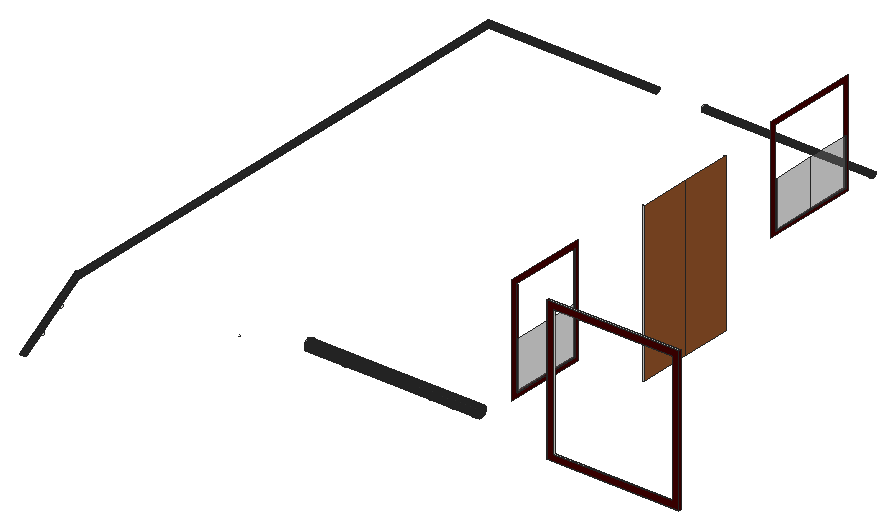
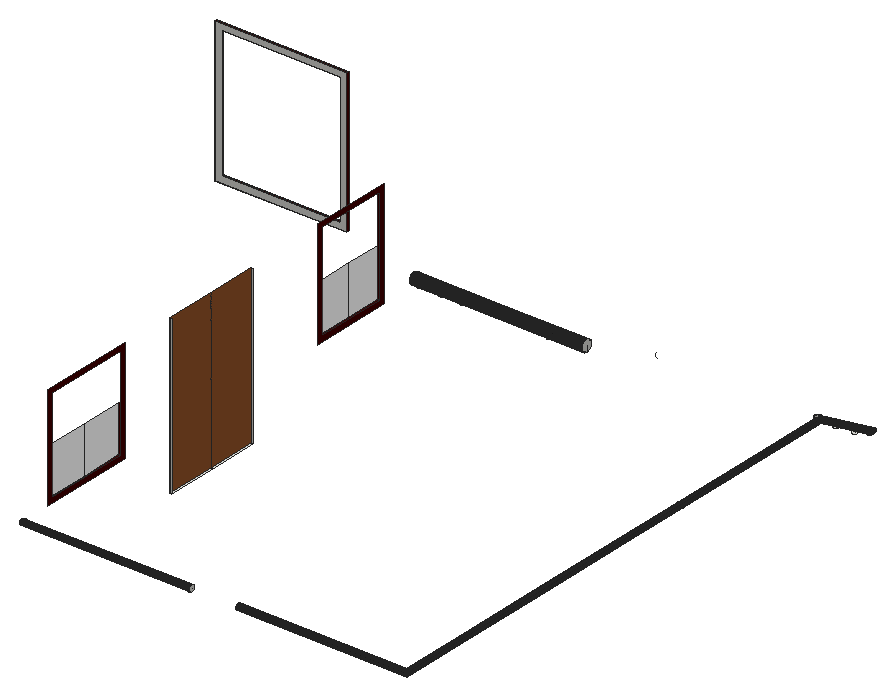
# SketchUp Ruby script. Lengths in inches.
U = 1.inch
M = Sketchup.active_model
def pt(a) = Geom::Point3d.new(a.map { |v| v * U })
def face(e, loops, mat)
  f = e.add_face(loops[0].map { |a| pt(a) })
  loops[1..].each { |l| e.add_face(l.map { |a| pt(a) }).erase! }
  f.material = f.back_material = mat if mat
  f
end
# faces: each face lists its corners as indices into pts; further lists are holes
def faces(e, pts, list, mat = nil) = list.each { |f| face(e, (f[0].is_a?(Array) ? f : [f]).map { |l| l.map { |i| pts[i] } }, mat) }
# xy, xz, yz: faces in a plane at the given z, y or x. An outline is a flat list of corners, or four numbers for a rectangle; further outlines are holes
def ring(l) = l.size == 4 ? [[l[0], l[1]], [l[2], l[1]], [l[2], l[3]], [l[0], l[3]]] : l.each_slice(2).to_a
def flat(e, list, mat, &to3) = list.each { |f| face(e, (f[0].is_a?(Array) ? f : [f]).map { |l| ring(l).map { |u, v| to3.(u, v) } }, mat) }
def xy(e, z, list, mat = nil) = flat(e, list, mat) { |x, y| [x, y, z] }
def xz(e, y, list, mat = nil) = flat(e, list, mat) { |x, z| [x, y, z] }
def yz(e, x, list, mat = nil) = flat(e, list, mat) { |y, z| [x, y, z] }
def lines(e, pts, list) = list.each { |a, b| e.add_line(pt(pts[a]), pt(pts[b])) }
# prism: a flat outline (further loops are holes) pulled along v
def prism(e, loops, v, mat = nil)
  f = face(e, loops, mat); d = Geom::Vector3d.new(v.map { |x| x * U })
  f.pushpull(f.normal.samedirection?(d) ? d.length : -d.length)
end
def box(e, o, s, mat = nil) = prism(e, [[o, [o[0] + s[0], o[1], o[2]], [o[0] + s[0], o[1] + s[1], o[2]], [o[0], o[1] + s[1], o[2]]]], [0, 0, s[2]], mat)
def at(x, y, z, deg = 0) = Geom::Transformation.translation(pt([x, y, z])) * Geom::Transformation.rotation(ORIGIN, Z_AXIS, deg.degrees)
def axes(o, x, y, z) = Geom::Transformation.new([*x, 0, *y, 0, *z, 0, *pt(o).to_a, 1])
def part(name) = M.definitions.add(name)
# library, detail: a bought-in or finely detailed component or shape, given as its bounding box
def library(name, o, s) = part(name).tap { |d| box(d.entities, o, s) }
def detail(e, o, s) = box(e.add_group.entities, o, s)
def put(e, d, t, mat = nil) = e.add_instance(d, t).tap { |i| i.material = mat if mat }
def group(e, t, mat = nil) = e.add_group.tap { |g| g.transformation = t; g.material = mat if mat }.entities
root = M.entities
M.materials.add("[0022_Maroon]").color = [68, 0, 0]
M.materials.add("[0137_Black]").color = [45, 45, 45]
M.materials.add("[Translucent Glass Gray]").color = [128, 128, 128]
M.materials["[Translucent Glass Gray]"].alpha = 0.5
M.materials.add("[Wood Cherry Original]").color = [152, 86, 42]
xy(root,53.06,[[432,334.98,434,391.49],[432,391.49,434,447.99]])
xy(root,82.48,[[4.7,30.03,5.01,30.03,5.33,30.07,5.63,30.14,5.93,30.24,6.22,30.37,6.49,30.53,6.74,30.72,6.97,30.93,7.18,31.17,7.36,31.42,7.51,31.7,7.64,31.98,7.73,32.28,7.79,32.59,7.82,32.9,7.82,33.22,7.78,33.53,7.71,33.84,7.61,34.13,7.48,34.42,7.32,34.6875,7.14,34.94,6.92,35.17,6.6875,35.38,6.43,35.5625,6.16,35.72,5.87,35.84,5.57,35.93,5.26,36,4.95,36.03,4.63,36.02,4.32,35.99,4.02,35.92,3.72,35.82,3.43,35.6875,3.16,35.53,2.91,35.34,2.68,35.125,2.47,34.89,2.29,34.63,2.14,34.36,2.01,34.07,1.92,33.77,1.86,33.46,1.83,33.15,1.83,32.84,1.87,32.53,1.9375,32.22,2.04,31.92,2.17,31.64,2.33,31.37,2.51,31.11,2.73,30.88,2.96,30.68,3.22,30.49,3.49,30.34,3.78,30.22,4.08,30.12,4.39,30.06]])
xy(root,98.83,[[5.56,55.09,5.875,55.09,6.1875,55.13,6.49,55.2,6.79,55.3,7.08,55.43,7.35,55.59,7.6,55.78,7.83,55.99,8.04,56.23,8.22,56.48,8.37,56.75,8.5,57.04,8.59,57.34,8.65,57.65,8.68,57.96,8.68,58.28,8.64,58.59,8.57,58.9,8.47,59.19,8.34,59.48,8.18,59.75,7.99,60,7.78,60.23,7.55,60.4375,7.29,60.62,7.02,60.78,6.73,60.9,6.43,60.99,6.12,61.06,5.81,61.08,5.49,61.08,5.18,61.05,4.875,60.98,4.58,60.875,4.29,60.75,4.02,60.59,3.77,60.4,3.54,60.19,3.33,59.95,3.15,59.69,3,59.42,2.87,59.13,2.78,58.83,2.72,58.52,2.6875,58.21,2.69,57.9,2.73,57.59,2.8,57.28,2.9,56.98,3.03,56.7,3.1875,56.43,3.375,56.17,3.59,55.94,3.82,55.74,4.08,55.55,4.35,55.4,4.64,55.27,4.94,55.18,5.25,55.12]])
xy(root,113.8,[[281.12,108.28,281.9,108.38,282.62,108.68,283.24,109.16,283.72,109.78,284.02,110.5,284.12,111.28,284.02,112.06,283.72,112.78,283.24,113.4,282.62,113.88,281.9,114.18,281.12,114.28,280.34,114.18,279.62,113.88,279,113.4,278.52,112.78,278.22,112.06,278.12,111.28,278.22,110.5,278.52,109.78,279,109.16,279.62,108.68,280.34,108.38]])
xy(root,114,[[377.12,108.28,376.34,108.38,375.62,108.68,375,109.16,374.52,109.78,374.22,110.5,374.12,111.28,380.12,111.28,380.02,110.5,379.72,109.78,379.24,109.16,378.62,108.68,377.9,108.38],[401.12,108.28,400.34,108.38,399.62,108.68,399,109.16,398.52,109.78,398.22,110.5,398.12,111.28,404.12,111.28,404.02,110.5,403.72,109.78,403.24,109.16,402.62,108.68,401.9,108.38],[425.12,108.28,424.34,108.38,423.62,108.68,423,109.16,422.52,109.78,422.22,110.5,422.12,111.28,428.12,111.28,428.02,110.5,427.72,109.78,427.24,109.16,426.62,108.68,425.9,108.38],[374.12,111.28,374.22,112.06,374.52,112.78,375,113.4,375.62,113.88,376.34,114.18,377.12,114.28,377.9,114.18,378.62,113.88,379.24,113.4,379.72,112.78,380.02,112.06,380.12,111.28],[398.12,111.28,398.22,112.06,398.52,112.78,399,113.4,399.62,113.88,400.34,114.18,401.12,114.28,401.9,114.18,402.62,113.88,403.24,113.4,403.72,112.78,404.02,112.06,404.12,111.28],
  [422.12,111.28,422.22,112.06,422.52,112.78,423,113.4,423.62,113.88,424.34,114.18,425.12,114.28,425.9,114.18,426.62,113.88,427.24,113.4,427.72,112.78,428.02,112.06,428.12,111.28]])
xy(root,118.5,[[432,159.23,434,238.92]],"[0022_Maroon]")
xy(root,119.9,[[528.3,82,674.74,84]])
xy(root,121.79,[[432,518.52,434,566.6875],[432,566.6875,434,614.85]],"[0022_Maroon]")
xz(root,82,[[[528.3,119.9,674.74,278.46],[535.0625,126.66,667.98,271.7]]],"[0022_Maroon]")
xz(root,84,[[[528.3,119.9,674.74,278.46],[535.0625,126.66,667.98,271.7]]])
xz(root,159.23,[[432,118.5,434,226.5]],"[0022_Maroon]")
xz(root,238.92,[[432,118.5,434,226.5]],"[0022_Maroon]")
xz(root,334.98,[[432,53.06,434,227.44]])
xz(root,447.99,[[432,53.06,434,227.44]])
xz(root,518.52,[[432,121.79,434,174.15]],"[0022_Maroon]")
xz(root,614.85,[[432,121.79,434,174.15]],"[0022_Maroon]")
yz(root,240,[[111.28,114,110.65,114.03,110.03,114.13,109.43,114.29,108.84,114.52,108.28,114.8,107.75,115.15,107.27,115.54,106.82,115.99,106.43,116.47,106.09,117,105.8,117.56,105.57,118.15,105.41,118.75,105.3125,119.37,105.28,120,105.3125,120.63,105.41,121.25,105.57,121.85,105.8,122.44,106.09,123,106.43,123.53,106.82,124.01,107.27,124.46,107.75,124.85,108.28,125.2,108.84,125.48,109.43,125.71,110.03,125.87,110.65,125.97,111.28,126,111.91,125.97,112.53,125.87,113.14,125.71,113.72,125.48,114.28,125.2,114.81,124.85,115.3,124.46,115.74,124.01,116.14,123.53,116.48,123,116.76,122.44,116.99,121.85,117.15,121.25,117.25,120.63,117.28,120,117.25,119.37,117.15,118.75,116.99,118.15,116.76,117.56,116.48,117,116.14,116.47,115.74,115.99,115.3,115.54,114.81,115.15,114.28,114.8,113.72,114.52,113.14,114.29,112.53,114.13,111.91,114.03]])
yz(root,243.11,[[655.94,113.61,655.17,113.71,654.44,114.01,653.82,114.49,653.34,115.11,653.04,115.83,652.94,116.61,653.04,117.39,653.34,118.11,653.82,118.73,654.44,119.21,655.17,119.51,655.94,119.61,656.72,119.51,657.44,119.21,658.0625,118.73,658.54,118.11,658.84,117.39,658.94,116.61,658.84,115.83,658.54,115.11,658.0625,114.49,657.44,114.01,656.72,113.71]])
yz(root,432,[[[153.23,112.5,244.92,232.5],[159.23,118.5,238.92,226.5]],[[513.28,116.55,620.09,231.74],[518.52,121.79,614.85,226.5]]],"[0022_Maroon]")
yz(root,434,[[159.23,118.5,199.08,172.5],[199.08,118.5,238.92,172.5],[518.52,121.79,566.6875,174.15],[566.6875,121.79,614.85,174.15]],"[Translucent Glass Gray]")
yz(root,434,[[[334.98,53.06,391.49,227.44],[383.84,140.25,385.71,163.32]],[[391.49,53.06,447.99,227.44],[397.59,140.25,399.46,163.32]]],"[Wood Cherry Original]")
yz(root,528.3,[[82,119.9,84,278.46]],"[0022_Maroon]")
yz(root,674.74,[[82,119.9,84,278.46]],"[0022_Maroon]")
p = [[4.82,11.11,70.34],[4.52,11.04,70.375],[4.2,87.78,117.04],[4.51,87.8125,116.98],[4.64,55.27,97.19],[5.13,11.15,70.32],
  [4.82,87.83,116.95],[5.45,11.15,70.31],[5.13,87.84,116.95],[5.76,11.12,70.33],[5.45,87.82,116.97],[6.07,11.0625,70.37],
  [5.75,87.79,117.03],[4.22,10.94,70.43],[3.93,10.8125,70.5],[3.62,87.66,117.23],[3.9,87.72,117.12],[6.66,10.84,70.49],
  [6.37,10.97,70.42],[6.1875,55.13,97.28],[6.05,87.74,117.11],[6.34,87.68,117.22],[3.66,10.65,70.59],[3.35,87.57,117.37],
  [6.93,10.6875,70.58],[6.61,87.6,117.35],[3.41,10.47,70.7],[3.09,87.47,117.53],[7.1875,10.51,70.68],[6.87,87.5,117.5],
  [3.18,10.25,70.82],[2.86,87.36,117.71],[7.42,10.3,70.8],[7.1,87.4,117.68],[2.97,10.02,70.95],[2.65,87.24,117.91],
  [7.63,10.07,70.93],[7.32,87.28,117.88],[2.79,9.76,71.09],[2.47,87.11,118.125],[7.82,9.82,71.07],[7.5,87.15,118.1],
  [2.64,9.49,71.24],[2.32,86.96,118.36],[7.98,9.55,71.22],[7.66,87.01,118.33],[2.51,9.2,71.41],[2.19,86.8125,118.61],
  [8.11,9.26,71.38],[7.79,86.86,118.57],[2.42,8.9,71.57],[2.1,86.66,118.86],[8.21,8.96,71.55],[7.89,86.7,118.83],
  [2.36,8.59,71.75],[2.04,86.5,119.125],[8.28,8.66,71.72],[7.96,86.54,119.09],[2.33,8.28,71.92],[2.01,86.34,119.39],
  [8.32,8.34,71.9],[8,86.38,119.36],[2.33,7.96,72.1],[2.01,86.17,119.66],[8.32,8.03,72.08],[8,86.22,119.625],
  [2.37,7.65,72.28],[2.04,86.01,119.93],[8.29,7.72,72.25],[7.97,86.06,119.89],[2.43,7.35,72.45],[2.11,85.85,120.1875],
  [8.23,7.41,72.43],[7.91,85.9,120.15],[2.53,7.05,72.62],[2.21,85.7,120.44],[8.14,7.11,72.59],[7.8125,85.74,120.41],
  [2.67,6.76,72.78],[2.34,85.55,120.6875],[8.01,6.82,72.76],[7.6875,85.59,120.66],[2.83,6.49,72.93],[2.5,85.41,120.92],
  [7.86,6.55,72.91],[7.53,85.45,120.89],[3.01,6.24,73.07],[2.6875,85.28,121.13],[7.68,6.29,73.05],[7.35,85.3125,121.11],
  [3.23,6.01,73.2],[2.9,85.16,121.33],[7.47,6.06,73.18],[7.14,85.19,121.31],[3.46,5.8,73.32],[3.14,85.05,121.51],
  [7.24,5.84,73.3],[6.91,85.08,121.49],[3.72,5.62,73.42],[3.39,84.96,121.67],[6.99,5.66,73.41],[6.66,84.98,121.65],
  [3.99,5.47,73.51],[3.67,84.88,121.8],[6.71,5.5,73.5],[6.39,84.9,121.78],[4.28,5.34,73.58],[3.95,84.8125,121.91],
  [6.43,5.37,73.57],[6.1,84.83,121.89],[4.58,5.25,73.63],[4.25,84.77,121.99],[4.89,5.1875,73.67],[4.56,84.73,122.04],
  [5.83,5.2,73.66],[6.13,5.27,73.625],[5.81,84.78,121.98],[5.5,84.74,122.04],[5.2,5.16,73.69],[4.87,84.72,122.07],
  [5.51,5.16,73.68],[5.1875,84.72,122.07],[3.45,275.17,113.71],[4.23,275.17,113.61],[4.23,269.37,113.61],[4.23,251.17,113.61],
  [4.23,245.37,113.61],[4.23,227.17,113.61],[4.23,221.37,113.61],[4.23,203.17,113.61],[4.23,197.37,113.61],[4.23,179.17,113.61],
  [4.23,173.37,113.61],[4.23,155.17,113.61],[4.23,149.37,113.61],[4.23,131.17,113.61],[4.23,125.37,113.61],[4.23,86.28,113.61],
  [3.45,86.28,113.71],[3.45,149.27,113.71],[3.45,155.27,113.71],[5,275.17,113.71],[5,269.27,113.71],[5,251.27,113.71],
  [5,245.27,113.71],[5,227.27,113.71],[5,221.27,113.71],[5,203.27,113.71],[5,197.27,113.71],[5,179.27,113.71],
  [5,173.27,113.71],[5,152.27,113.71],[5,131.27,113.71],[5,125.27,113.71],[5,86.28,113.71],[3.45,464.06,113.71],
  [4.23,464.06,113.61],[4.23,458.26,113.61],[4.23,440.06,113.61],[4.23,434.26,113.61],[4.23,416.06,113.61],[4.23,410.26,113.61],
  [4.23,392.06,113.61],[4.23,386.26,113.61],[4.23,368.06,113.61],[4.23,362.26,113.61],[4.23,344.06,113.61],[4.23,338.26,113.61],
  [4.23,320.06,113.61],[4.23,314.26,113.61],[3.45,338.16,113.71],[3.45,344.16,113.71],[5,464.06,113.71],[5,458.16,113.71],
  [5,440.16,113.71],[5,434.16,113.71],[5,416.16,113.71],[5,410.16,113.71],[5,392.16,113.71],[5,386.16,113.71],
  [5,368.16,113.71],[5,362.16,113.71],[5,341.16,113.71],[5,320.16,113.71],[5,314.16,113.71],[5,275.27,113.71],
  [3.45,652.94,113.71],[4.23,652.94,113.61],[4.23,647.15,113.61],[4.23,628.94,113.61],[4.23,623.15,113.61],[4.23,604.94,113.61],
  [4.23,599.15,113.61],[4.23,580.94,113.61],[4.23,575.15,113.61],[4.23,556.94,113.61],[4.23,551.15,113.61],[4.23,532.94,113.61],
  [4.23,527.15,113.61],[4.23,508.94,113.61],[4.23,503.15,113.61],[3.45,527.05,113.71],[3.45,533.05,113.71],[5,652.94,113.71],
  [5,647.05,113.71],[5,629.05,113.71],[5,623.05,113.71],[5,605.05,113.71],[5,599.05,113.71],[5,581.05,113.71],
  [5,575.05,113.71],[5,557.05,113.71],[5,551.05,113.71],[5,530.05,113.71],[5,509.05,113.71],[5,503.05,113.71],
  [5,464.16,113.71],[2.74,655.17,113.71],[2.74,655.94,113.61],[8.53,655.94,113.61],[26.74,655.94,113.61],[32.53,655.94,113.61],
  [50.74,655.94,113.61],[56.53,655.94,113.61],[74.74,655.94,113.61],[80.53,655.94,113.61],[98.74,655.94,113.61],[104.53,655.94,113.61],
  [122.74,655.94,113.61],[128.53,655.94,113.61],[146.74,655.94,113.61],[152.53,655.94,113.61],[191.625,655.94,113.61],[191.625,655.17,113.71],
  [128.63,655.17,113.71],[122.63,655.17,113.71],[243.11,655.17,113.71],[243.11,655.94,113.61],[248.91,655.94,113.61],[267.11,655.94,113.61],
  [272.91,655.94,113.61],[291.11,655.94,113.61],[296.91,655.94,113.61],[315.11,655.94,113.61],[320.91,655.94,113.61],[339.11,655.94,113.61],
  [344.91,655.94,113.61],[363.11,655.94,113.61],[368.91,655.94,113.61],[387.11,655.94,113.61],[392.91,655.94,113.61],[432,655.94,113.61],
  [432,655.17,113.71],[369.01,655.17,113.71],[363.01,655.17,113.71],[2.74,656.72,113.71],[8.63,656.72,113.71],[26.63,656.72,113.71],
  [32.63,656.72,113.71],[50.63,656.72,113.71],[56.63,656.72,113.71],[74.63,656.72,113.71],[80.63,656.72,113.71],[98.63,656.72,113.71],
  [104.63,656.72,113.71],[125.63,656.72,113.71],[146.63,656.72,113.71],[152.63,656.72,113.71],[191.625,656.72,113.71],[243.11,656.72,113.71],
  [249.01,656.72,113.71],[267.01,656.72,113.71],[273.01,656.72,113.71],[291.01,656.72,113.71],[297.01,656.72,113.71],[315.01,656.72,113.71],
  [321.01,656.72,113.71],[339.01,656.72,113.71],[345.01,656.72,113.71],[366.01,656.72,113.71],[387.01,656.72,113.71],[393.01,656.72,113.71],
  [432,656.72,113.71],[2.73,275.17,114.01],[2.73,86.28,114.01],[5.73,275.17,114.01],[5.73,86.28,114.01],[2.73,464.06,114.01],
  [5.73,464.06,114.01],[2.73,652.94,114.01],[5.73,652.94,114.01],[2.74,654.44,114.01],[191.625,654.44,114.01],[243.11,654.44,114.01],
  [432,654.44,114.01],[2.74,657.44,114.01],[191.625,657.44,114.01],[243.11,657.44,114.01],[432,657.44,114.01],[2.11,275.17,114.49],
  [2.11,86.28,114.49],[6.35,275.17,114.49],[6.35,86.28,114.49],[240,110.03,114.13],[240,110.65,114.03],[432,110.65,114.03],
  [432,110.03,114.13],[240,111.28,114],[257.12,111.28,114],[281.12,111.28,114],[305.12,111.28,114],[329.12,111.28,114],
  [353.12,111.28,114],[374.12,111.28,114],[377.12,111.28,114],[380.12,111.28,114],[398.12,111.28,114],[401.12,111.28,114],
  [404.12,111.28,114],[422.12,111.28,114],[425.12,111.28,114],[428.12,111.28,114],[432,111.28,114],[240,111.91,114.03],
  [432,111.91,114.03],[240,112.53,114.13],[432,112.53,114.13],[2.11,464.06,114.49],[6.35,464.06,114.49],[2.11,652.94,114.49],
  [6.35,652.94,114.49],[2.74,653.82,114.49],[191.625,653.82,114.49],[243.11,653.82,114.49],[432,653.82,114.49],[2.74,658.0625,114.49],
  [191.625,658.0625,114.49],[243.11,658.0625,114.49],[432,658.0625,114.49],[240,109.43,114.29],[432,109.43,114.29],[240,113.14,114.29],
  [432,113.14,114.29],[240,108.84,114.52],[432,108.84,114.52],[240,113.72,114.52],[432,113.72,114.52],[1.63,275.17,115.11],
  [1.63,86.28,115.11],[6.82,275.17,115.11],[6.82,86.28,115.11],[240,108.28,114.8],[432,108.28,114.8],[240,114.28,114.8],
  [432,114.28,114.8],[1.63,464.06,115.11],[6.82,464.06,115.11],[1.63,652.94,115.11],[6.82,652.94,115.11],[2.74,653.34,115.11],
  [191.625,653.34,115.11],[243.11,653.34,115.11],[432,653.34,115.11],[2.74,658.54,115.11],[191.625,658.54,115.11],[243.11,658.54,115.11],
  [432,658.54,115.11],[240,107.75,115.15],[432,107.75,115.15],[240,114.81,115.15],[432,114.81,115.15],[1.33,275.17,115.83],
  [1.33,86.28,115.83],[7.125,275.17,115.83],[7.125,86.28,115.83],[240,107.27,115.54],[432,107.27,115.54],[240,115.3,115.54],
  [432,115.3,115.54],[1.33,464.06,115.83],[7.125,464.06,115.83],[1.33,652.94,115.83],[7.125,652.94,115.83],[2.74,653.04,115.83],
  [191.625,653.04,115.83],[243.11,653.04,115.83],[432,653.04,115.83],[2.74,658.84,115.83],[191.625,658.84,115.83],[243.11,658.84,115.83],
  [432,658.84,115.83],[240,106.82,115.99],[432,106.82,115.99],[240,115.74,115.99],[432,115.74,115.99],[1.23,275.17,116.61],
  [1.23,86.28,116.61],[7.23,275.17,116.61],[7.23,86.28,116.61],[1.23,464.06,116.61],[7.23,464.06,116.61],[1.23,652.94,116.61],
  [7.23,652.94,116.61],[2.74,652.94,116.61],[191.625,652.94,116.61],[243.11,652.94,116.61],[432,652.94,116.61],[2.74,658.94,116.61],
  [191.625,658.94,116.61],[243.11,658.94,116.61],[432,658.94,116.61],[240,106.43,116.47],[432,106.43,116.47],[240,116.14,116.47],
  [432,116.14,116.47],[240,106.09,117],[432,106.09,117],[240,116.48,117],[432,116.48,117],[1.33,275.17,117.39],
  [1.33,86.28,117.39],[7.125,275.17,117.39],[7.125,86.28,117.39],[1.33,464.06,117.39],[7.125,464.06,117.39],[1.33,652.94,117.39],
  [7.125,652.94,117.39],[2.74,653.04,117.39],[191.625,653.04,117.39],[243.11,653.04,117.39],[432,653.04,117.39],[2.74,658.84,117.39],
  [191.625,658.84,117.39],[243.11,658.84,117.39],[432,658.84,117.39],[240,105.8,117.56],[432,105.8,117.56],[240,116.76,117.56],
  [432,116.76,117.56],[1.63,275.17,118.11],[1.63,86.28,118.11],[6.82,275.17,118.11],[6.82,86.28,118.11],[1.63,464.06,118.11],
  [6.82,464.06,118.11],[1.63,652.94,118.11],[6.82,652.94,118.11],[2.74,653.34,118.11],[191.625,653.34,118.11],[243.11,653.34,118.11],
  [432,653.34,118.11],[2.74,658.54,118.11],[191.625,658.54,118.11],[243.11,658.54,118.11],[432,658.54,118.11],[240,105.57,118.15],
  [432,105.57,118.15],[240,116.99,118.15],[432,116.99,118.15],[2.11,275.17,118.73],[2.11,86.28,118.73],[6.35,275.17,118.73],
  [6.35,86.28,118.73],[240,105.41,118.75],[432,105.41,118.75],[240,117.15,118.75],[432,117.15,118.75],[2.11,464.06,118.73],
  [6.35,464.06,118.73],[2.11,652.94,118.73],[6.35,652.94,118.73],[2.74,653.82,118.73],[191.625,653.82,118.73],[243.11,653.82,118.73],
  [432,653.82,118.73],[2.74,658.0625,118.73],[191.625,658.0625,118.73],[243.11,658.0625,118.73],[432,658.0625,118.73],[2.73,275.17,119.21],
  [2.73,86.28,119.21],[5.73,275.17,119.21],[5.73,86.28,119.21],[2.73,464.06,119.21],[5.73,464.06,119.21],[2.73,652.94,119.21],
  [5.73,652.94,119.21],[2.74,654.44,119.21],[191.625,654.44,119.21],[243.11,654.44,119.21],[432,654.44,119.21],[2.74,657.44,119.21],
  [191.625,657.44,119.21],[243.11,657.44,119.21],[432,657.44,119.21],[240,105.3125,119.37],[432,105.3125,119.37],[240,117.25,119.37],
  [432,117.25,119.37],[3.45,275.17,119.51],[3.45,86.28,119.51],[5,275.17,119.51],[5,86.28,119.51],[3.45,464.06,119.51],
  [5,464.06,119.51],[3.45,652.94,119.51],[5,652.94,119.51],[2.74,655.17,119.51],[191.625,655.17,119.51],[243.11,655.17,119.51],
  [432,655.17,119.51],[2.74,656.72,119.51],[191.625,656.72,119.51],[243.11,656.72,119.51],[432,656.72,119.51],[240,105.28,120],
  [432,105.28,120],[240,117.28,120],[432,117.28,120],[4.23,275.17,119.61],[4.23,86.28,119.61],[4.23,464.06,119.61],
  [4.23,652.94,119.61],[2.74,655.94,119.61],[191.625,655.94,119.61],[243.11,655.94,119.61],[432,655.94,119.61],[240,105.3125,120.63],
  [432,105.3125,120.63],[240,117.25,120.63],[432,117.25,120.63],[240,105.41,121.25],[432,105.41,121.25],[240,117.15,121.25],
  [432,117.15,121.25],[240,105.57,121.85],[432,105.57,121.85],[240,116.99,121.85],[432,116.99,121.85],[240,105.8,122.44],
  [432,105.8,122.44],[240,116.76,122.44],[432,116.76,122.44],[240,106.09,123],[432,106.09,123],[240,116.48,123],
  [432,116.48,123],[240,106.43,123.53],[432,106.43,123.53],[240,116.14,123.53],[432,116.14,123.53],[240,106.82,124.01],
  [432,106.82,124.01],[240,115.74,124.01],[432,115.74,124.01],[240,107.27,124.46],[432,107.27,124.46],[240,115.3,124.46],
  [432,115.3,124.46],[240,107.75,124.85],[432,107.75,124.85],[240,114.81,124.85],[432,114.81,124.85],[240,108.28,125.2],
  [432,108.28,125.2],[240,114.28,125.2],[432,114.28,125.2],[240,108.84,125.48],[432,108.84,125.48],[240,113.72,125.48],
  [432,113.72,125.48],[240,109.43,125.71],[432,109.43,125.71],[240,113.14,125.71],[432,113.14,125.71],[240,110.03,125.87],
  [432,110.03,125.87],[240,112.53,125.87],[432,112.53,125.87],[240,110.65,125.97],[432,110.65,125.97],[240,111.91,125.97],
  [432,111.91,125.97],[240,111.28,126],[432,111.28,126],[432,111.28,120],[240,111.28,120],[257.12,111.28,113.58],
  [281.12,111.28,113.8],[305.12,111.28,113.8],[243.11,655.94,116.61],[432,655.94,116.61],[366.01,656.72,114],[5.32,8.15,72],
  [4.82,33.03,82.48],[4.82,33.03,83.45],[4.82,33.03,83.625],[183.77,84.89,121.9],[184.12,85.18,121.26],[184.27,85.51,120.5625],
  [184.21,85.85,119.86],[183.96,86.17,119.19],[183.52,86.47,118.61],[182.93,86.71,118.16],[182.23,86.88,117.86],[181.46,86.98,117.74]]
faces(root,p,[[0,1,2,3,4],[5,0,4,3,6],[7,5,6,8],[9,7,8,10],[11,9,10,12],[13,14,15,16],[17,18,19,20,21],[1,13,16,2],
  [18,11,12,20,19],[14,22,23,15],[24,17,21,25],[22,26,27,23],[28,24,25,29],[26,30,31,27],[32,28,29,33],[30,34,35,31],
  [36,32,33,37],[34,38,39,35],[40,36,37,41],[38,42,43,39],[44,40,41,45],[42,46,47,43],[48,44,45,49],[46,50,51,47],
  [52,48,49,53],[50,54,55,51],[56,52,53,57],[54,58,59,55],[60,56,57,61],[58,62,63,59],[64,60,61,65],[62,66,67,63],
  [68,64,65,69],[66,70,71,67],[72,68,69,73],[70,74,75,71],[76,72,73,77],[74,78,79,75],[80,76,77,81],[78,82,83,79],
  [84,80,81,85],[82,86,87,83],[88,84,85,89],[86,90,91,87],[92,88,89,93],[90,94,95,91],[96,92,93,97],[94,98,99,95],
  [100,96,97,101],[98,102,103,99],[104,100,101,105],[102,106,107,103],[108,104,105,109],[106,110,111,107],[110,112,113,111],[114,115,116,117],
  [115,108,109,116],[112,118,119,113],[118,120,121,119],[120,114,117,121],[122,123,124,125,126,127,128,129,130,131,132,133,134,135,136,137,138,139,140],[123,141,142,143,144,145,146,147,148,149,150,151,152,153,154,137,136,135,134,133,132,131,130,129,128,127,126,125,124],[155,156,157,158,159,160,161,162,163,164,165,166,167,168,169,123,122,170,171],[156,172,173,174,175,176,177,178,179,180,181,182,183,184,185,141,123,169,168,167,166,165,164,163,162,161,160,159,158,157],
  [186,187,188,189,190,191,192,193,194,195,196,197,198,199,200,156,155,201,202],[187,203,204,205,206,207,208,209,210,211,212,213,214,215,216,172,156,200,199,198,197,196,195,194,193,192,191,190,189,188],[217,218,219,220,221,222,223,224,225,226,227,228,229,230,231,232,233,234,235],[236,237,238,239,240,241,242,243,244,245,246,247,248,249,250,251,252,253,254],[218,255,256,257,258,259,260,261,262,263,264,265,266,267,268,232,231,230,229,228,227,226,225,224,223,222,221,220,219],[237,269,270,271,272,273,274,275,276,277,278,279,280,281,282,251,250,249,248,247,246,245,244,243,242,241,240,239,238],[283,122,140,139,138,284],[141,285,286,154,153,152,151,150,149,148,147,146,145,144,143,142],
  [287,155,171,170,122,283],[172,288,285,141,185,184,183,182,181,180,179,178,177,176,175,174,173],[289,186,202,201,155,287],[203,290,288,172,216,215,214,213,212,211,210,209,208,207,206,205,204],[291,217,235,234,233,292],[293,236,254,253,252,294],[255,295,296,268,267,266,265,264,263,262,261,260,259,258,257,256],[269,297,298,282,281,280,279,278,277,276,275,274,273,272,271,270],
  [299,283,284,300],[285,301,302,286],[303,304,305,306],[304,307,308,309,310,311,312,313,314,315,316,317,318,319,320,321,322,305],[307,323,324,322,321,320,319,318,317,316,315,314,313,312,311,310,309,308],[323,325,326,324],[327,287,283,299],[288,328,301,285],
  [329,289,287,327],[290,330,328,288],[331,291,292,332],[333,293,294,334],[295,335,336,296],[297,337,338,298],[339,303,306,340],[325,341,342,326],
  [343,339,340,344],[341,345,346,342],[347,299,300,348],[301,349,350,302],[351,343,344,352],[345,353,354,346],[355,327,299,347],[328,356,349,301],
  [357,329,327,355],[330,358,356,328],[359,331,332,360],[361,333,334,362],[335,363,364,336],[337,365,366,338],[367,351,352,368],[353,369,370,354],
  [371,347,348,372],[349,373,374,350],[375,367,368,376],[369,377,378,370],[379,355,347,371],[356,380,373,349],[381,357,355,379],[358,382,380,356],
  [383,359,360,384],[385,361,362,386],[363,387,388,364],[365,389,390,366],[391,375,376,392],[377,393,394,378],[395,371,372,396],[373,397,398,374],
  [399,379,371,395],[380,400,397,373],[401,381,379,399],[382,402,400,380],[403,383,384,404],[405,385,386,406],[387,407,408,388],[389,409,410,390],
  [411,391,392,412],[393,413,414,394],[415,411,412,416],[413,417,418,414],[419,395,396,420],[397,421,422,398],[423,399,395,419],[400,424,421,397],
  [425,401,399,423],[402,426,424,400],[427,403,404,428],[429,405,406,430],[407,431,432,408],[409,433,434,410],[435,415,416,436],[417,437,438,418],
  [439,419,420,440],[421,441,442,422],[443,423,419,439],[424,444,441,421],[445,425,423,443],[426,446,444,424],[447,427,428,448],[449,429,430,450],
  [431,451,452,432],[433,453,454,434],[455,435,436,456],[437,457,458,438],[459,439,440,460],[441,461,462,442],[463,455,456,464],[457,465,466,458],
  [467,443,439,459],[444,468,461,441],[469,445,443,467],[446,470,468,444],[471,447,448,472],[473,449,450,474],[451,475,476,452],[453,477,478,454],
  [479,459,460,480],[461,481,482,462],[483,467,459,479],[468,484,481,461],[485,469,467,483],[470,486,484,468],[487,471,472,488],[489,473,474,490],
  [475,491,492,476],[477,493,494,478],[495,463,464,496],[465,497,498,466],[499,479,480,500],[481,501,502,482],[503,483,479,499],[484,504,501,481],
  [505,485,483,503],[486,506,504,484],[507,487,488,508],[509,489,490,510],[491,511,512,492],[493,513,514,494],[515,495,496,516],[497,517,518,498],
  [519,499,500,520],[501,519,520,502],[521,503,499,519],[504,521,519,501],[522,505,503,521],[506,522,521,504],[523,507,508,524],[525,509,510,526],
  [511,523,524,512],[513,525,526,514],[527,515,516,528],[517,529,530,518],[531,527,528,532],[529,533,534,530],[535,531,532,536],[533,537,538,534],
  [539,535,536,540],[537,541,542,538],[543,539,540,544],[541,545,546,542],[547,543,544,548],[545,549,550,546],[551,547,548,552],[549,553,554,550],
  [555,551,552,556],[553,557,558,554],[559,555,556,560],[557,561,562,558],[563,559,560,564],[561,565,566,562],[567,563,564,568],[565,569,570,566],
  [571,567,568,572],[569,573,574,570],[575,571,572,576],[573,577,578,574],[579,575,576,580],[577,581,582,578],[583,579,580,584],[581,583,584,582]],"[0137_Black]")
faces(root,p,[[41,37,33,29,25,21,20,12,10,8,6,3,2,16,15,23,27,31,35,39,43,47,51,55,59,63,67,71,75,79,83,87,91,95,99,103,107,111,113,119,121,117,116,109,105,101,97,93,89,85,81,77,73,69,65,61,57,53,49,45]])
lines(root,p,[[585,586],[586,307],[322,585],[587,308],[588,309],[589,310],[590,591],[279,592],[593,502],[594,595],[595,596],[597,598],
  [598,599],[599,600],[600,601],[601,602],[602,603],[603,604],[604,605]])
